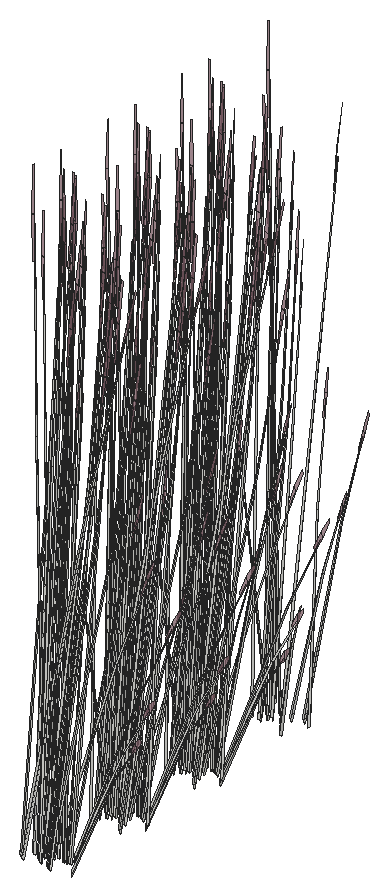
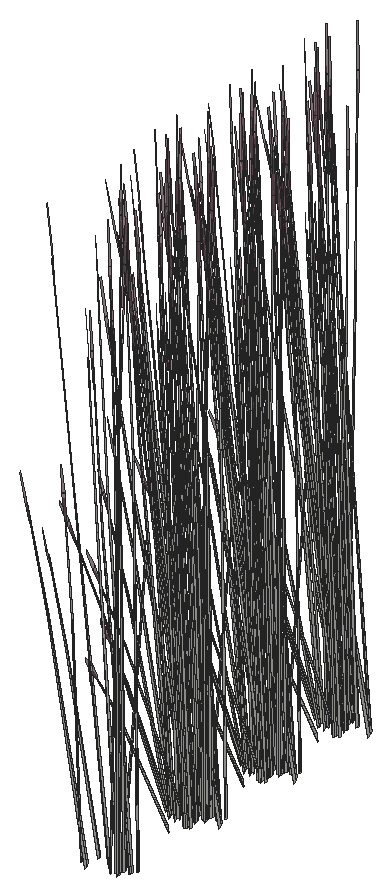
# SketchUp Ruby script. Lengths in inches.
U = 1.inch
M = Sketchup.active_model
def pt(a) = Geom::Point3d.new(a.map { |v| v * U })
def face(e, loops, mat)
  f = e.add_face(loops[0].map { |a| pt(a) })
  loops[1..].each { |l| e.add_face(l.map { |a| pt(a) }).erase! }
  f.material = f.back_material = mat if mat
  f
end
# faces: each face lists its corners as indices into pts; further lists are holes
def faces(e, pts, list, mat = nil) = list.each { |f| face(e, (f[0].is_a?(Array) ? f : [f]).map { |l| l.map { |i| pts[i] } }, mat) }
# xy, xz, yz: faces in a plane at the given z, y or x. An outline is a flat list of corners, or four numbers for a rectangle; further outlines are holes
def ring(l) = l.size == 4 ? [[l[0], l[1]], [l[2], l[1]], [l[2], l[3]], [l[0], l[3]]] : l.each_slice(2).to_a
def flat(e, list, mat, &to3) = list.each { |f| face(e, (f[0].is_a?(Array) ? f : [f]).map { |l| ring(l).map { |u, v| to3.(u, v) } }, mat) }
def xy(e, z, list, mat = nil) = flat(e, list, mat) { |x, y| [x, y, z] }
def xz(e, y, list, mat = nil) = flat(e, list, mat) { |x, z| [x, y, z] }
def yz(e, x, list, mat = nil) = flat(e, list, mat) { |y, z| [x, y, z] }
def lines(e, pts, list) = list.each { |a, b| e.add_line(pt(pts[a]), pt(pts[b])) }
# prism: a flat outline (further loops are holes) pulled along v
def prism(e, loops, v, mat = nil)
  f = face(e, loops, mat); d = Geom::Vector3d.new(v.map { |x| x * U })
  f.pushpull(f.normal.samedirection?(d) ? d.length : -d.length)
end
def box(e, o, s, mat = nil) = prism(e, [[o, [o[0] + s[0], o[1], o[2]], [o[0] + s[0], o[1] + s[1], o[2]], [o[0], o[1] + s[1], o[2]]]], [0, 0, s[2]], mat)
def at(x, y, z, deg = 0) = Geom::Transformation.translation(pt([x, y, z])) * Geom::Transformation.rotation(ORIGIN, Z_AXIS, deg.degrees)
def axes(o, x, y, z) = Geom::Transformation.new([*x, 0, *y, 0, *z, 0, *pt(o).to_a, 1])
def part(name) = M.definitions.add(name)
# library, detail: a bought-in or finely detailed component or shape, given as its bounding box
def library(name, o, s) = part(name).tap { |d| box(d.entities, o, s) }
def detail(e, o, s) = box(e.add_group.entities, o, s)
def put(e, d, t, mat = nil) = e.add_instance(d, t).tap { |i| i.material = mat if mat }
def group(e, t, mat = nil) = e.add_group.tap { |g| g.transformation = t; g.material = mat if mat }.entities
root = M.entities
M.materials.add("LightPink_Translucent").color = [144, 107, 117]
M.materials["LightPink_Translucent"].alpha = 0.75
c1 = part("blade")
p = [[2.15,0.21,22],[0,0.17,0],[0.09,0.45,0],[2.18,0.31,22],[2.29,0.31,22],[0.38,0.45,0],
  [2.48,0.24,33],[2.49,0.24,33],[2.48,0.22,33]]
faces(c1.entities,p,[[0,1,2,3],[4,5,2,3],[6,3,4,7],[8,0,3,6]])
c2 = part("seeds")
p = [[0.3,-0.1,1.38],[-0.01,-0.03,1.59],[-0.01,-0.03,0.03],[0.14,-0.07,-0.07],[0.29,-0.03,3],[0.15,0.01,3.11]]
faces(c2.entities,p,[[0,1,2,3],[1,0,4,5]],"LightPink_Translucent")
c3 = part("blade with seeds")
put(c3.entities,c1,at(0,0,0))
put(c3.entities,c2,axes([2.4,0.25,30.99],[1.5799,-0.05474,1.17369],[-0.12525,1.92788,0.29478],[-0.07173,-0.02425,1.56792]))
put(root,c3,axes([334.21,396.62,49.95],[0,-0.45213,0],[0.63136,0,0],[0,0,1.58567]))
put(root,c3,axes([334.97,395.57,50.19],[-0.47255,-0.19538,0.43871],[0.28245,-0.35034,0],[0.10763,0.0445,1.3917]))
put(root,c3,axes([333.91,396.33,50.09],[-0.41865,0.35461,0.40429],[-0.49737,-0.31303,0.15865],[0.10093,-0.03539,1.40366]))
put(root,c3,axes([333.18,395.75,50.1875],[-0.14586,0.38834,0.15589],[-0.53375,-0.1099,0.31002],[0.0922,-0.00189,1.41735]))
put(root,c3,axes([332.96,396.0625,49.41],[-0.49699,0.15644,1.13921],[-0.15819,-0.44887,0.44265],[0.30518,0.00747,1.29573]))
put(root,c3,axes([334.29,396.18,50.3125],[0.09741,-0.34873,0.12794],[0.4759,0.06053,-0.36534],[0.08661,0.03581,1.11991]))
put(root,c3,axes([336.84,396.67,49.32],[-0.02639,-0.05932,1.55816],[0.18302,-0.34702,-0.23804],[0.18462,-0.00499,0.26541]))
put(root,c3,axes([334.09,396.27,50.4],[-0.30332,-0.32798,0.39531],[0.45944,-0.23096,-0.19025],[0.09816,0.04058,1.26923]))
put(root,c3,axes([334.25,396.3,50.36],[0.50979,-0.25942,-0.25709],[0.339,0.36656,-0.44182],[0.12578,0.03723,1.41118]))
put(root,c3,axes([335.53,395.61,49.78],[0.47255,0.19538,-0.43871],[-0.28245,0.35034,0],[0.10763,0.0445,1.3917]))
put(root,c3,axes([334.63,396.72,49.95],[0.56491,0,0],[0,0.40454,0],[0,0,1.5764]))
put(root,c3,axes([334.79,395.77,50.1875],[-0.54257,0.10371,0.15589],[-0.13397,-0.38597,0.31002],[0.04839,0.05624,1.41735]))
put(root,c3,axes([335.4,395.75,49.79],[0.11861,0.34048,-0.27372],[-0.47106,0.09668,0.27372],[0.09497,0.03926,1.22797]))
put(root,c3,axes([334.45,396.51,50.1],[-0.63817,-0.08233,0.43472],[0.12987,-0.46497,0.17059],[0.09326,0.0449,1.50931]))
put(root,c3,axes([334.56,397.62,49.93],[0.53009,-0.13258,-0.16963],[0.18627,0.38191,0.00007],[0.05851,-0.01465,1.53656]))
put(root,c3,axes([334.62,396.89,49.96],[0.35245,0.2524,0],[-0.35245,0.2524,0],[0,0,1.49564]))
put(root,c3,axes([335.58,396.78,50.1875],[-0.39671,-0.28463,0.15589],[0.39978,-0.27607,0.31002],[-0.04381,0.05813,1.41735]))
put(root,c3,axes([334.84,396.35,49.82],[0.52523,0.06406,-0.55095],[-0.11084,0.39517,-0.1446],[0.15674,0.04788,1.21613]))
put(root,c3,axes([334.62,396.6,50.4],[0.24498,-0.3521,0.39531],[0.50902,0.16945,-0.19025],[0,0.08116,1.26923]))
put(root,c3,axes([334.52,396.8,50.03],[0,0.45191,-0.04981],[-0.63136,0,0],[0,0.0142,1.58489]))
put(root,c3,axes([334.57,396.48,49.95],[0.30332,0.32798,-0.39531],[-0.45944,0.23096,0.19025],[0.09816,0.04058,1.26923]))
put(root,c3,axes([335.9,396.8,50.19],[0,-0.39075,0.43871],[0.56491,0,0],[0,0.089,1.3917]))
put(root,c3,axes([334.83,396.68,50.3125],[0.47043,-0.11396,0.12794],[0.16474,0.32541,-0.36534],[0,0.07162,1.11991]))
put(root,c3,axes([336.58,397.47,50.29],[-0.1216,-0.0961,1.26356],[0.15822,-0.31792,-0.27174],[0.24603,0.04307,0.54024]))
put(root,c3,axes([334.4,397.82,49.95],[0.50902,0.17543,0],[-0.24498,0.36452,0],[0,0,1.54589]))
put(root,c3,axes([334.22,397.67,50.02],[0.21952,0.44891,-0.05313],[-0.62724,0.1573,0],[0.00767,0.01568,1.52132]))
put(root,c3,axes([336.29,396.86,50.1],[0.63136,0,0],[0,0.43672,-0.456],[0,0.09947,1.44655]))
put(root,c3,axes([336.03,397.09,49.94],[-0.63105,-0.00312,-0.04397],[0,-0.43672,0.44129],[-0.01983,0.09942,1.3992]))
put(root,c3,axes([334.67,396.71,50.36],[0.56863,0.18645,-0.25709],[-0.2738,0.39352,-0.44182],[0.01787,0.09662,1.41118]))
put(root,c3,axes([335.9,397.15,49.79],[-0.35245,0.2438,-0.27372],[-0.35245,-0.2438,0.27372],[0,0.07853,1.22797]))
put(root,c3,axes([334.61,397,49.95],[-0.24498,0.3521,-0.39531],[-0.50902,-0.16945,0.19025],[0,0.08116,1.26923]))
put(root,c3,axes([336.15,397.16,49.78],[0,0.39075,-0.43871],[-0.56491,0,0],[0,0.089,1.3917]))
put(root,c3,axes([335.51,398.39,49.32],[0.03679,-0.05641,1.55816],[0.46313,-0.16615,-0.23804],[0.14041,0.08599,0.26541]))
put(root,c3,axes([334.9,397.1,49.85],[0.18514,0.35777,-0.61156],[-0.53331,0.12885,-0.16051],[0.02046,0.12115,1.3499]))
put(root,c3,axes([335.47,398.48,50.36],[-0.32378,-0.01225,0.92831],[0.21383,-0.26028,0.51254],[0.12791,0.09247,0.72818]))
put(root,c3,axes([334.77,403.42,50.29],[-0.14352,0.07909,1.26356],[-0.42983,-0.13843,-0.27174],[0.07968,-0.17216,0.54024]))
put(root,c3,axes([334.42,397.85,50.29],[0.00891,-0.12953,1.26356],[0.4258,-0.14469,-0.27174],[0.13144,0.15503,0.54024]))
put(root,c3,axes([335.77,403.66,49.32],[-0.07557,-0.03078,1.55816],[-0.19412,-0.34391,-0.23804],[0.13095,-0.09333,0.26541]))
put(root,c3,axes([332.92,403.73,50.1],[-0.31568,-0.39156,0],[0.52815,-0.21836,-0.456],[0.12029,-0.04973,1.44655]))
put(root,c3,axes([333.35,403.67,49.78],[0.47255,-0.19538,-0.43871],[0.28245,0.35034,0],[0.10763,-0.0445,1.3917]))
put(root,c3,axes([336.15,404.35,50.29],[-0.18038,-0.01157,1.26356],[-0.18479,-0.31048,-0.27174],[0.22159,-0.08783,0.54024]))
put(root,c3,axes([333.91,404.47,49.82],[0.34009,-0.2937,-0.55095],[0.42248,0.26632,-0.1446],[0.13628,-0.07327,1.21613]))
put(root,c3,axes([333.54,404.8125,50.36],[-0.05884,-0.44587,-0.25709],[0.6128,-0.02696,-0.44182],[0.10791,-0.05939,1.41118]))
put(root,c3,axes([333.46,403.83,49.79],[0.47106,0.09668,-0.27372],[-0.11861,0.34048,0.27372],[0.09497,-0.03926,1.22797]))
put(root,c3,axes([333.62,405.16,50.15],[0.56891,0.18939,0.21263],[-0.2738,0.39352,0.44182],[0,-0.09071,1.41855]))
put(root,c3,axes([333.44,404.9,50.4],[-0.54829,0.02412,0.39531],[-0.04958,-0.40041,-0.19025],[0.09816,-0.04058,1.26923]))
put(root,c3,axes([335.24,403.83,50.1],[0.31568,-0.39156,0],[0.52815,0.21836,-0.456],[0.12029,0.04973,1.44655]))
put(root,c3,axes([336.49,405.38,49.75],[-0.3252,0.04689,1.25103],[-0.05176,-0.37326,0.07161],[0.22777,-0.0565,0.71188]))
put(root,c3,axes([337.08,405.05,50],[-0.31304,-0.24986,-0.05733],[0.34284,-0.22894,-0.25992],[0.09714,-0.01612,0.85731]))
put(root,c3,axes([334.21,405.08,49.95],[0,-0.45213,0],[0.63136,0,0],[0,0,1.58567]))
put(root,c3,axes([334.97,404.04,50.19],[-0.47255,-0.19538,0.43871],[0.28245,-0.35034,0],[0.10763,0.0445,1.3917]))
put(root,c3,axes([333.91,404.8,50.09],[-0.41865,0.35461,0.40429],[-0.49737,-0.31303,0.15865],[0.10093,-0.03539,1.40366]))
put(root,c3,axes([333.18,404.21,50.1875],[-0.14586,0.38834,0.15589],[-0.53375,-0.1099,0.31002],[0.0922,-0.00189,1.41735]))
put(root,c3,axes([332.96,404.53,49.41],[-0.49699,0.15644,1.13921],[-0.15819,-0.44887,0.44265],[0.30518,0.00747,1.29573]))
put(root,c3,axes([334.29,404.64,50.3125],[0.09741,-0.34873,0.12794],[0.4759,0.06053,-0.36534],[0.08661,0.03581,1.11991]))
put(root,c3,axes([336.84,405.14,49.32],[-0.02639,-0.05932,1.55816],[0.18302,-0.34702,-0.23804],[0.18462,-0.00499,0.26541]))
put(root,c3,axes([334.09,404.74,50.4],[-0.30332,-0.32798,0.39531],[0.45944,-0.23096,-0.19025],[0.09816,0.04058,1.26923]))
put(root,c3,axes([334.25,404.76,50.36],[0.50979,-0.25942,-0.25709],[0.339,0.36656,-0.44182],[0.12578,0.03723,1.41118]))
put(root,c3,axes([335.53,404.07,49.78],[0.47255,0.19538,-0.43871],[-0.28245,0.35034,0],[0.10763,0.0445,1.3917]))
put(root,c3,axes([334.63,405.18,49.95],[0.56491,0,0],[0,0.40454,0],[0,0,1.5764]))
put(root,c3,axes([334.79,404.23,50.1875],[-0.54257,0.10371,0.15589],[-0.13397,-0.38597,0.31002],[0.04839,0.05624,1.41735]))
put(root,c3,axes([335.4,404.21,49.79],[0.11861,0.34048,-0.27372],[-0.47106,0.09668,0.27372],[0.09497,0.03926,1.22797]))
put(root,c3,axes([334.45,404.98,50.1],[-0.63817,-0.08233,0.43472],[0.12987,-0.46497,0.17059],[0.09326,0.0449,1.50931]))
put(root,c3,axes([334.56,406.08,49.93],[0.53009,-0.13258,-0.16963],[0.18627,0.38191,0.00007],[0.05851,-0.01465,1.53656]))
put(root,c3,axes([334.62,405.36,49.96],[0.35245,0.2524,0],[-0.35245,0.2524,0],[0,0,1.49564]))
put(root,c3,axes([335.58,405.25,50.1875],[-0.39671,-0.28463,0.15589],[0.39978,-0.27607,0.31002],[-0.04381,0.05813,1.41735]))
put(root,c3,axes([334.84,404.82,49.82],[0.52523,0.06406,-0.55095],[-0.11084,0.39517,-0.1446],[0.15674,0.04788,1.21613]))
put(root,c3,axes([334.62,405.06,50.4],[0.24498,-0.3521,0.39531],[0.50902,0.16945,-0.19025],[0,0.08116,1.26923]))
put(root,c3,axes([334.52,405.26,50.03],[0,0.45191,-0.04981],[-0.63136,0,0],[0,0.0142,1.58489]))
put(root,c3,axes([334.57,404.94,49.95],[0.30332,0.32798,-0.39531],[-0.45944,0.23096,0.19025],[0.09816,0.04058,1.26923]))
put(root,c3,axes([335.9,405.26,50.19],[0,-0.39075,0.43871],[0.56491,0,0],[0,0.089,1.3917]))
put(root,c3,axes([334.83,405.14,50.3125],[0.47043,-0.11396,0.12794],[0.16474,0.32541,-0.36534],[0,0.07162,1.11991]))
put(root,c3,axes([336.58,405.93,50.29],[-0.1216,-0.0961,1.26356],[0.15822,-0.31792,-0.27174],[0.24603,0.04307,0.54024]))
put(root,c3,axes([334.4,406.28,49.95],[0.50902,0.17543,0],[-0.24498,0.36452,0],[0,0,1.54589]))
put(root,c3,axes([334.22,406.14,50.02],[0.21952,0.44891,-0.05313],[-0.62724,0.1573,0],[0.00767,0.01568,1.52132]))
put(root,c3,axes([336.29,405.32,50.1],[0.63136,0,0],[0,0.43672,-0.456],[0,0.09947,1.44655]))
put(root,c3,axes([336.03,405.55,49.94],[-0.63105,-0.00312,-0.04397],[0,-0.43672,0.44129],[-0.01983,0.09942,1.3992]))
put(root,c3,axes([334.67,405.17,50.36],[0.56863,0.18645,-0.25709],[-0.2738,0.39352,-0.44182],[0.01787,0.09662,1.41118]))
put(root,c3,axes([335.9,405.61,49.79],[-0.35245,0.2438,-0.27372],[-0.35245,-0.2438,0.27372],[0,0.07853,1.22797]))
put(root,c3,axes([334.61,405.46,49.95],[-0.24498,0.3521,-0.39531],[-0.50902,-0.16945,0.19025],[0,0.08116,1.26923]))
put(root,c3,axes([336.15,405.62,49.78],[0,0.39075,-0.43871],[-0.56491,0,0],[0,0.089,1.3917]))
put(root,c3,axes([335.51,406.85,49.32],[0.03679,-0.05641,1.55816],[0.46313,-0.16615,-0.23804],[0.14041,0.08599,0.26541]))
put(root,c3,axes([334.9,405.57,49.85],[0.18514,0.35777,-0.61156],[-0.53331,0.12885,-0.16051],[0.02046,0.12115,1.3499]))
put(root,c3,axes([335.47,406.94,50.36],[-0.32378,-0.01225,0.92831],[0.21383,-0.26028,0.51254],[0.12791,0.09247,0.72818]))
put(root,c3,axes([334.77,411.88,50.29],[-0.14352,0.07909,1.26356],[-0.42983,-0.13843,-0.27174],[0.07968,-0.17216,0.54024]))
put(root,c3,axes([334.42,406.31,50.29],[0.00891,-0.12953,1.26356],[0.4258,-0.14469,-0.27174],[0.13144,0.15503,0.54024]))
put(root,c3,axes([335.77,412.125,49.32],[-0.07557,-0.03078,1.55816],[-0.19412,-0.34391,-0.23804],[0.13095,-0.09333,0.26541]))
put(root,c3,axes([332.92,412.2,50.1],[-0.31568,-0.39156,0],[0.52815,-0.21836,-0.456],[0.12029,-0.04973,1.44655]))
put(root,c3,axes([333.35,412.14,49.78],[0.47255,-0.19538,-0.43871],[0.28245,0.35034,0],[0.10763,-0.0445,1.3917]))
put(root,c3,axes([336.15,412.8125,50.29],[-0.18038,-0.01157,1.26356],[-0.18479,-0.31048,-0.27174],[0.22159,-0.08783,0.54024]))
put(root,c3,axes([333.91,412.94,49.82],[0.34009,-0.2937,-0.55095],[0.42248,0.26632,-0.1446],[0.13628,-0.07327,1.21613]))
put(root,c3,axes([333.54,413.28,50.36],[-0.05884,-0.44587,-0.25709],[0.6128,-0.02696,-0.44182],[0.10791,-0.05939,1.41118]))
put(root,c3,axes([333.46,412.29,49.79],[0.47106,0.09668,-0.27372],[-0.11861,0.34048,0.27372],[0.09497,-0.03926,1.22797]))
put(root,c3,axes([333.62,413.63,50.15],[0.56891,0.18939,0.21263],[-0.2738,0.39352,0.44182],[0,-0.09071,1.41855]))
put(root,c3,axes([333.44,413.37,50.4],[-0.54829,0.02412,0.39531],[-0.04958,-0.40041,-0.19025],[0.09816,-0.04058,1.26923]))
put(root,c3,axes([335.24,412.3,50.1],[0.31568,-0.39156,0],[0.52815,0.21836,-0.456],[0.12029,0.04973,1.44655]))
put(root,c3,axes([336.49,413.85,49.75],[-0.3252,0.04689,1.25103],[-0.05176,-0.37326,0.07161],[0.22777,-0.0565,0.71188]))
put(root,c3,axes([337.08,413.51,50],[-0.31304,-0.24986,-0.05733],[0.34284,-0.22894,-0.25992],[0.09714,-0.01612,0.85731]))
put(root,c3,axes([334.21,413.55,49.95],[0,-0.45213,0],[0.63136,0,0],[0,0,1.58567]))
put(root,c3,axes([334.97,412.5,50.19],[-0.47255,-0.19538,0.43871],[0.28245,-0.35034,0],[0.10763,0.0445,1.3917]))
put(root,c3,axes([333.91,413.26,50.09],[-0.41865,0.35461,0.40429],[-0.49737,-0.31303,0.15865],[0.10093,-0.03539,1.40366]))
put(root,c3,axes([333.18,412.68,50.1875],[-0.14586,0.38834,0.15589],[-0.53375,-0.1099,0.31002],[0.0922,-0.00189,1.41735]))
put(root,c3,axes([332.96,412.99,49.41],[-0.49699,0.15644,1.13921],[-0.15819,-0.44887,0.44265],[0.30518,0.00747,1.29573]))
put(root,c3,axes([334.29,413.11,50.3125],[0.09741,-0.34873,0.12794],[0.4759,0.06053,-0.36534],[0.08661,0.03581,1.11991]))
put(root,c3,axes([336.84,413.6,49.32],[-0.02639,-0.05932,1.55816],[0.18302,-0.34702,-0.23804],[0.18462,-0.00499,0.26541]))
put(root,c3,axes([334.09,413.2,50.4],[-0.30332,-0.32798,0.39531],[0.45944,-0.23096,-0.19025],[0.09816,0.04058,1.26923]))
put(root,c3,axes([334.25,413.22,50.36],[0.50979,-0.25942,-0.25709],[0.339,0.36656,-0.44182],[0.12578,0.03723,1.41118]))
put(root,c3,axes([335.53,412.53,49.78],[0.47255,0.19538,-0.43871],[-0.28245,0.35034,0],[0.10763,0.0445,1.3917]))
put(root,c3,axes([334.63,413.65,49.95],[0.56491,0,0],[0,0.40454,0],[0,0,1.5764]))
put(root,c3,axes([334.79,412.7,50.1875],[-0.54257,0.10371,0.15589],[-0.13397,-0.38597,0.31002],[0.04839,0.05624,1.41735]))
put(root,c3,axes([335.4,412.68,49.79],[0.11861,0.34048,-0.27372],[-0.47106,0.09668,0.27372],[0.09497,0.03926,1.22797]))
put(root,c3,axes([334.45,413.44,50.1],[-0.63817,-0.08233,0.43472],[0.12987,-0.46497,0.17059],[0.09326,0.0449,1.50931]))
put(root,c3,axes([334.56,414.54,49.93],[0.53009,-0.13258,-0.16963],[0.18627,0.38191,0.00007],[0.05851,-0.01465,1.53656]))
put(root,c3,axes([334.62,413.82,49.96],[0.35245,0.2524,0],[-0.35245,0.2524,0],[0,0,1.49564]))
put(root,c3,axes([335.58,413.71,50.1875],[-0.39671,-0.28463,0.15589],[0.39978,-0.27607,0.31002],[-0.04381,0.05813,1.41735]))
put(root,c3,axes([334.84,413.28,49.82],[0.52523,0.06406,-0.55095],[-0.11084,0.39517,-0.1446],[0.15674,0.04788,1.21613]))
put(root,c3,axes([334.62,413.53,50.4],[0.24498,-0.3521,0.39531],[0.50902,0.16945,-0.19025],[0,0.08116,1.26923]))
put(root,c3,axes([334.52,413.73,50.03],[0,0.45191,-0.04981],[-0.63136,0,0],[0,0.0142,1.58489]))
put(root,c3,axes([334.57,413.41,49.95],[0.30332,0.32798,-0.39531],[-0.45944,0.23096,0.19025],[0.09816,0.04058,1.26923]))
put(root,c3,axes([335.9,413.72,50.19],[0,-0.39075,0.43871],[0.56491,0,0],[0,0.089,1.3917]))
put(root,c3,axes([334.83,413.61,50.3125],[0.47043,-0.11396,0.12794],[0.16474,0.32541,-0.36534],[0,0.07162,1.11991]))
put(root,c3,axes([336.58,414.4,50.29],[-0.1216,-0.0961,1.26356],[0.15822,-0.31792,-0.27174],[0.24603,0.04307,0.54024]))
put(root,c3,axes([334.4,414.75,49.95],[0.50902,0.17543,0],[-0.24498,0.36452,0],[0,0,1.54589]))
put(root,c3,axes([334.22,414.6,50.02],[0.21952,0.44891,-0.05313],[-0.62724,0.1573,0],[0.00767,0.01568,1.52132]))
put(root,c3,axes([336.29,413.79,50.1],[0.63136,0,0],[0,0.43672,-0.456],[0,0.09947,1.44655]))
put(root,c3,axes([336.03,414.01,49.94],[-0.63105,-0.00312,-0.04397],[0,-0.43672,0.44129],[-0.01983,0.09942,1.3992]))
put(root,c3,axes([334.67,413.63,50.36],[0.56863,0.18645,-0.25709],[-0.2738,0.39352,-0.44182],[0.01787,0.09662,1.41118]))
put(root,c3,axes([335.9,414.08,49.79],[-0.35245,0.2438,-0.27372],[-0.35245,-0.2438,0.27372],[0,0.07853,1.22797]))
put(root,c3,axes([334.61,413.93,49.95],[-0.24498,0.3521,-0.39531],[-0.50902,-0.16945,0.19025],[0,0.08116,1.26923]))
put(root,c3,axes([336.15,414.09,49.78],[0,0.39075,-0.43871],[-0.56491,0,0],[0,0.089,1.3917]))
put(root,c3,axes([335.51,415.3125,49.32],[0.03679,-0.05641,1.55816],[0.46313,-0.16615,-0.23804],[0.14041,0.08599,0.26541]))
put(root,c3,axes([334.9,414.03,49.85],[0.18514,0.35777,-0.61156],[-0.53331,0.12885,-0.16051],[0.02046,0.12115,1.3499]))
put(root,c3,axes([335.47,415.41,50.36],[-0.32378,-0.01225,0.92831],[0.21383,-0.26028,0.51254],[0.12791,0.09247,0.72818]))
put(root,c3,axes([334.42,414.78,50.29],[0.00891,-0.12953,1.26356],[0.4258,-0.14469,-0.27174],[0.13144,0.15503,0.54024]))
put(root,c3,axes([334.77,421.78,50.29],[-0.14352,0.07909,1.26356],[-0.42983,-0.13843,-0.27174],[0.07968,-0.17216,0.54024]))
put(root,c3,axes([335.77,422.02,49.32],[-0.07557,-0.03078,1.55816],[-0.19412,-0.34391,-0.23804],[0.13095,-0.09333,0.26541]))
put(root,c3,axes([332.92,422.1,50.1],[-0.31568,-0.39156,0],[0.52815,-0.21836,-0.456],[0.12029,-0.04973,1.44655]))
put(root,c3,axes([333.35,422.04,49.78],[0.47255,-0.19538,-0.43871],[0.28245,0.35034,0],[0.10763,-0.0445,1.3917]))
put(root,c3,axes([336.15,422.71,50.29],[-0.18038,-0.01157,1.26356],[-0.18479,-0.31048,-0.27174],[0.22159,-0.08783,0.54024]))
put(root,c3,axes([333.91,422.84,49.82],[0.34009,-0.2937,-0.55095],[0.42248,0.26632,-0.1446],[0.13628,-0.07327,1.21613]))
put(root,c3,axes([333.54,423.18,50.36],[-0.05884,-0.44587,-0.25709],[0.6128,-0.02696,-0.44182],[0.10791,-0.05939,1.41118]))
put(root,c3,axes([333.46,422.19,49.79],[0.47106,0.09668,-0.27372],[-0.11861,0.34048,0.27372],[0.09497,-0.03926,1.22797]))
put(root,c3,axes([333.62,423.53,50.15],[0.56891,0.18939,0.21263],[-0.2738,0.39352,0.44182],[0,-0.09071,1.41855]))
put(root,c3,axes([333.44,423.26,50.4],[-0.54829,0.02412,0.39531],[-0.04958,-0.40041,-0.19025],[0.09816,-0.04058,1.26923]))
put(root,c3,axes([335.24,422.2,50.1],[0.31568,-0.39156,0],[0.52815,0.21836,-0.456],[0.12029,0.04973,1.44655]))
put(root,c3,axes([336.49,423.74,49.75],[-0.3252,0.04689,1.25103],[-0.05176,-0.37326,0.07161],[0.22777,-0.0565,0.71188]))
put(root,c3,axes([337.08,423.41,50],[-0.31304,-0.24986,-0.05733],[0.34284,-0.22894,-0.25992],[0.09714,-0.01612,0.85731]))
put(root,c3,axes([334.21,423.44,49.95],[0,-0.45213,0],[0.63136,0,0],[0,0,1.58567]))
